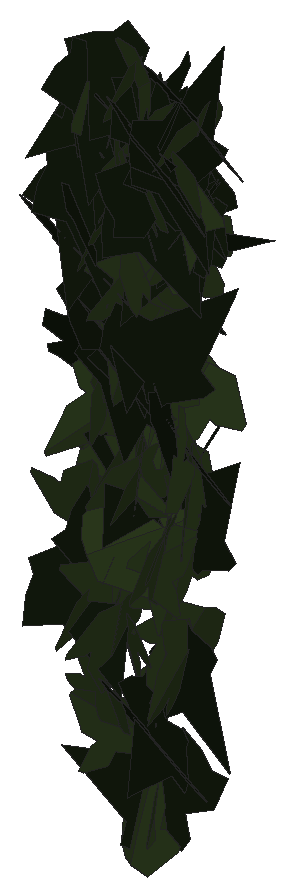
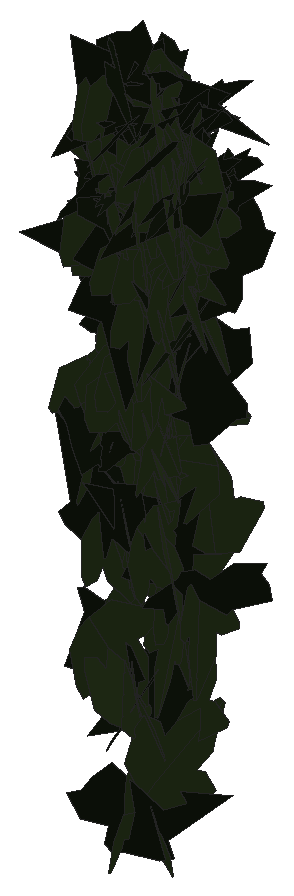
# SketchUp Ruby script. Lengths in inches.
U = 1.inch
M = Sketchup.active_model
def pt(a) = Geom::Point3d.new(a.map { |v| v * U })
def face(e, loops, mat)
  f = e.add_face(loops[0].map { |a| pt(a) })
  loops[1..].each { |l| e.add_face(l.map { |a| pt(a) }).erase! }
  f.material = f.back_material = mat if mat
  f
end
# faces: each face lists its corners as indices into pts; further lists are holes
def faces(e, pts, list, mat = nil) = list.each { |f| face(e, (f[0].is_a?(Array) ? f : [f]).map { |l| l.map { |i| pts[i] } }, mat) }
# xy, xz, yz: faces in a plane at the given z, y or x. An outline is a flat list of corners, or four numbers for a rectangle; further outlines are holes
def ring(l) = l.size == 4 ? [[l[0], l[1]], [l[2], l[1]], [l[2], l[3]], [l[0], l[3]]] : l.each_slice(2).to_a
def flat(e, list, mat, &to3) = list.each { |f| face(e, (f[0].is_a?(Array) ? f : [f]).map { |l| ring(l).map { |u, v| to3.(u, v) } }, mat) }
def xy(e, z, list, mat = nil) = flat(e, list, mat) { |x, y| [x, y, z] }
def xz(e, y, list, mat = nil) = flat(e, list, mat) { |x, z| [x, y, z] }
def yz(e, x, list, mat = nil) = flat(e, list, mat) { |y, z| [x, y, z] }
def lines(e, pts, list) = list.each { |a, b| e.add_line(pt(pts[a]), pt(pts[b])) }
# prism: a flat outline (further loops are holes) pulled along v
def prism(e, loops, v, mat = nil)
  f = face(e, loops, mat); d = Geom::Vector3d.new(v.map { |x| x * U })
  f.pushpull(f.normal.samedirection?(d) ? d.length : -d.length)
end
def box(e, o, s, mat = nil) = prism(e, [[o, [o[0] + s[0], o[1], o[2]], [o[0] + s[0], o[1] + s[1], o[2]], [o[0], o[1] + s[1], o[2]]]], [0, 0, s[2]], mat)
def at(x, y, z, deg = 0) = Geom::Transformation.translation(pt([x, y, z])) * Geom::Transformation.rotation(ORIGIN, Z_AXIS, deg.degrees)
def axes(o, x, y, z) = Geom::Transformation.new([*x, 0, *y, 0, *z, 0, *pt(o).to_a, 1])
def part(name) = M.definitions.add(name)
# library, detail: a bought-in or finely detailed component or shape, given as its bounding box
def library(name, o, s) = part(name).tap { |d| box(d.entities, o, s) }
def detail(e, o, s) = box(e.add_group.entities, o, s)
def put(e, d, t, mat = nil) = e.add_instance(d, t).tap { |i| i.material = mat if mat }
def group(e, t, mat = nil) = e.add_group.tap { |g| g.transformation = t; g.material = mat if mat }.entities
root = M.entities
M.materials.add("efeu1").color = [18, 25, 13]
M.materials.add("efeu2").color = [43, 57, 29]
c1 = part("ivyleaf_9")
p = [[1.54,2.16,1.25],[1.36,2.04,1.19],[-0.21,0.99,0.68],[-0.71,1.11,0.82],[-0.85,0.86,0.67],[-0.8,0.17,0.21],
  [-0.9,-0.01,0.1],[-0.67,-0.16,-0.02],[-0.08,-0.08,-0.05],[-0.03,-0.6,-0.4],[0.65,-0.88,-0.66],[0.83,-0.6,-0.49],
  [1.29,-0.42,-0.43],[1.8125,-0.07,-0.26],[1.21,0.44,0.15]]
faces(c1.entities,p,[[0,1,2,3,4,5,6,7,8,9,10,11,12,13,14]],"efeu1")
c2 = part("ivyleaf_10")
p = [[0,0.5,-0.03],[-0.0625,2.02,-0.43],[-0.19,2.01,-0.46],[-0.54,1.05,-0.29],[-0.52,0.625,-0.18],[-0.83,0.76,-0.28],
  [-1.16,0.64,-0.33],[-1.15,0.33,-0.24],[-0.77,-0.39,0.02],[-0.3,-0.51,0.16],[0.04,-0.48,0.23],[-0.02,2.01,-0.4375],
  [-0.06,2.01,-0.43],[0.04,-0.49,0.23],[0.67,-0.49,0.14],[1.38,0.36,-0.2],[1.375,0.51,-0.24],[0.81,0.65,-0.19],
  [0.62,0.59,-0.15],[0.6,1.09,-0.28],[0.5,1.23,-0.31]]
faces(c2.entities,p,[[0,1,2,3,4,5,6,7,8,9,10],[11,12,0,13,14,15,16,17,18,19,20]],"efeu2")
put(root,c1,axes([25.3,224.21,220.79],[0.23727,-0.27625,0.34262],[0.27235,-0.2136,-0.36083],[0.34573,0.35785,0.04911]))
put(root,c2,axes([25.7,224.74,222.02],[0.25708,-0.41846,-0.09381],[0.00924,0.11476,-0.48656],[0.42874,0.24844,0.06674]))
put(root,c2,axes([25.66,224.67,221.51],[0.33755,0.36179,-0.07186],[-0.05541,-0.04658,-0.49473],[-0.36468,0.34196,0.00865]))
put(root,c2,axes([25.78,224.24,216.53],[0.03843,-0.45656,-0.20019],[-0.0113,0.19994,-0.45815],[0.49839,0.03974,0.00505]))
put(root,c2,axes([25.7,224.72,222.3],[-0.4666,-0.11612,-0.13712],[0.13863,0.01007,-0.48029],[0.1143,-0.48623,0.0228]))
put(root,c1,axes([25.71,223.97,221.64],[0.35482,-0.12342,-0.32996],[-0.28859,0.16676,-0.37271],[0.20204,0.45493,0.04711]))
put(root,c2,axes([25.67,224.15,217.47],[-0.46983,-0.00104,0.17107],[0.17106,-0.00683,0.46978],[0.00136,0.49995,0.00677]))
put(root,c2,axes([25.91,224.8,214.64],[-0.20183,-0.25034,-0.38287],[-0.23596,-0.30154,0.32155],[-0.3919,0.31048,0.00358]))
put(root,c2,axes([25.84,224.67,221.86],[-0.18116,-0.46591,-0.01034],[0.00679,0.00846,-0.49988],[0.46598,-0.18125,0.00326]))
put(root,c1,axes([25.38,224.33,219.46],[0.38974,-0.04686,0.30968],[0.30851,-0.02792,-0.39249],[0.05407,0.49702,0.00715]))
put(root,c2,axes([25.94,224.21,220.41],[0.34987,-0.21771,-0.28319],[-0.23378,0.16016,-0.41194],[0.27007,0.42066,0.01028]))
put(root,c2,axes([25.81,224.68,221.92],[0.16857,-0.46716,0.05788],[0.0158,-0.05583,-0.49662],[0.47046,0.16926,-0.00405]))
put(root,c1,axes([25.57,224.5625,222.11],[0.49853,0.03827,0],[-0.00502,0.0654,-0.49568],[-0.03794,0.49423,0.06559]))
put(root,c1,axes([25.67,224.74,221.89],[0.01646,-0.49973,-0.00146],[0.00007,0.00146,-0.5],[0.49973,0.01646,0.00011]))
put(root,c1,axes([25.77,224.4,221.54],[-0.1775,-0.46732,0.01028],[-0.00411,-0.00944,-0.49989],[0.46742,-0.17755,-0.00049]))
put(root,c2,axes([26.0625,224.37,220.65],[0.23074,-0.22348,-0.38316],[-0.28403,0.25731,-0.32112],[0.34071,0.36585,-0.00821]))
put(root,c1,axes([25.69,224.21,216.82],[-0.06647,-0.41296,-0.27395],[0.05339,0.26882,-0.41819],[0.49268,-0.08485,0.00836]))
put(root,c2,axes([25.81,224.6875,221.76],[-0.46903,-0.09695,-0.14357],[0.14605,0.00158,-0.47819],[0.09317,-0.49051,0.02684]))
put(root,c2,axes([25.77,224.73,221.42],[-0.3733,-0.28773,-0.16692],[0.2134,-0.01468,-0.45194],[0.25517,-0.40865,0.13376]))
put(root,c2,axes([25.6875,224.45,222.45],[0.11924,-0.43016,0.22526],[0.26979,-0.13417,-0.39901],[0.40372,0.21671,0.20011]))
put(root,c2,axes([25.84,224.52,222.52],[0.34144,-0.35958,0.06418],[0.03602,-0.05428,-0.49574],[0.36348,0.34315,-0.01116]))
put(root,c2,axes([25.85,224.91,218.9375],[-0.10473,0.40267,-0.27729],[-0.02921,-0.28823,-0.40752],[-0.48803,-0.06916,0.0839]))
put(root,c1,axes([25.77,224.59,222.75],[-0.08731,-0.4881,0.0643],[0.00023,-0.06534,-0.49571],[0.49232,-0.08653,0.01164]))
put(root,c2,axes([26.02,224.23,215.18],[-0.45975,0.17524,-0.08898],[-0.08678,0.02211,0.49191],[0.17634,0.46776,0.01009]))
put(root,c1,axes([25.6,224.75,222.06],[0.33348,-0.37031,0.04079],[0.05507,-0.00514,-0.49693],[0.36846,0.33592,0.03736]))
put(root,c2,axes([25.95,224.71,222.12],[-0.23348,-0.43652,-0.07027],[0.03089,0.06316,-0.49503],[0.44106,-0.23551,-0.00252]))
put(root,c1,axes([26.13,224.52,222.92],[-0.47502,-0.12045,0.09924],[-0.08474,-0.06791,-0.48806],[0.13106,-0.4805,0.0441]))
put(root,c2,axes([25.99,224.74,220.95],[-0.31643,-0.3736,0.10147],[0.01272,-0.14101,-0.47954],[0.38692,-0.3009,0.09874]))
put(root,c2,axes([25.9,224.59,222.18],[-0.37426,0.32688,-0.05548],[0.0445,-0.03339,-0.4969],[-0.32856,-0.37687,-0.0041]))
put(root,c1,axes([25.79,224.23,221.74],[0.00212,-0.49178,-0.09024],[0.0083,0.09027,-0.49171],[0.49993,0.00059,0.00854]))
put(root,c2,axes([26.03,224.46,216.28],[-0.39846,0.27118,0.133],[-0.10656,0.0798,-0.48195],[-0.28262,-0.41242,-0.0058]))
put(root,c2,axes([26.03,224.61,219.26],[0.05715,0.38173,-0.31783],[-0.17546,-0.28378,-0.3724],[-0.4647,0.1541,0.10153]))
put(root,c2,axes([26.04,224.16,221.4],[0.13555,-0.44192,-0.19062],[-0.06145,0.18052,-0.46221],[0.47734,0.14873,-0.00537]))
put(root,c2,axes([25.875,224.69,220.625],[-0.07184,-0.32443,0.37361],[0.19061,-0.36654,-0.28164],[0.45663,0.10196,0.17634]))
put(root,c1,axes([25.75,224.66,222.44],[0.16645,-0.44634,-0.15191],[0.00711,0.16346,-0.47247],[0.47143,0.15513,0.06077]))
put(root,c2,axes([26.15,224.31,219.05],[-0.13075,-0.18535,0.44559],[-0.1311,-0.43065,-0.2176],[0.46445,-0.17374,0.06402]))
put(root,c2,axes([26.02,224.66,220.2],[0.31523,-0.38728,-0.02535],[-0.01406,0.02123,-0.49935],[0.38786,0.31553,0.00249]))
put(root,c2,axes([26.29,224.14,221.51],[0.18426,-0.04059,-0.46303],[-0.36484,0.29598,-0.17113],[0.28799,0.40093,0.07946]))
put(root,c2,axes([26.03,224.14,219.34],[0.14162,-0.36303,-0.31329],[0.04213,0.33482,-0.36894],[0.47767,0.0781,0.12542]))
put(root,c2,axes([26.12,224.42,217.4375],[0.19341,-0.43236,-0.16017],[-0.07627,0.1413,-0.47352],[0.45473,0.2076,-0.01129]))
put(root,c1,axes([25.79,224.65,219.99],[0.17145,-0.44736,0.1431],[0.06303,-0.12904,-0.47893],[0.46544,0.18226,0.01214]))
put(root,c2,axes([26.0625,224.58,222.9],[0.1817,-0.4647,0.03219],[0.03058,-0.02258,-0.49855],[0.46481,0.18314,0.02022]))
put(root,c2,axes([26.05,224.74,218.85],[0.26099,-0.41098,0.11391],[0.05113,-0.10243,-0.48672],[0.4234,0.26571,-0.01144]))
put(root,c2,axes([26.28,224.39,222.93],[0.25108,-0.19096,-0.38794],[-0.26478,0.28675,-0.31252],[0.34184,0.36237,0.04287]))
put(root,c1,axes([26.08,224.65,222.53],[-0.25924,-0.42666,-0.02758],[0.01099,0.0256,-0.49922],[0.42741,-0.25944,-0.0039]))
put(root,c1,axes([25.86,224.02,220.27],[0.34819,-0.35427,-0.05709],[-0.0222,0.05813,-0.49611],[0.35815,0.34801,0.02475]))
put(root,c2,axes([26.18,224.82,220.94],[-0.40043,-0.28659,0.08674],[0.02348,-0.17444,-0.468],[0.2985,-0.37073,0.15316]))
put(root,c2,axes([26.17,224.73,220.29],[-0.09299,-0.47939,-0.10743],[0.01803,0.10593,-0.48832],[0.49095,-0.09469,-0.00241]))
put(root,c2,axes([25.89,224.58,221.36],[0.35948,0.13645,-0.31962],[0.28213,0.15392,0.38303],[0.20292,-0.45573,0.03367]))
put(root,c2,axes([26.17,224.76,221.61],[0.17502,-0.45573,-0.10809],[0.0004,0.11553,-0.48647],[0.46837,0.17019,0.04081]))
put(root,c2,axes([26.31,224.91,219.25],[-0.45041,-0.10275,0.19125],[-0.13178,-0.22064,-0.4289],[0.17254,-0.43676,0.17167]))
put(root,c1,axes([26.51,224.85,213.83],[-0.09773,0.04002,0.48872],[-0.48866,0.03351,-0.10046],[-0.04079,-0.49727,0.03257]))
put(root,c2,axes([26.1,224.76,217.41],[0.0094,-0.39176,0.31055],[0.13132,-0.29776,-0.3796],[0.48235,0.0887,0.09729]))
put(root,c2,axes([26.1,224.38,222.39],[-0.15869,0.45616,-0.12936],[0.01757,-0.13066,-0.48231],[-0.47382,-0.15762,0.02544]))
put(root,c2,axes([26.21,224.09,216.4375],[-0.01514,-0.4997,-0.00823],[0.00519,0.00808,-0.49991],[0.49974,-0.01522,0.00495]))
put(root,c2,axes([26.31,224.51,222.06],[-0.39405,-0.29531,0.08671],[-0.0673,-0.05479,-0.49241],[0.30033,-0.39974,0.00343]))
put(root,c2,axes([26.21,224.21,216.74],[-0.41114,-0.27656,0.0669],[0.05589,0.03678,0.4955],[-0.279,0.41492,0.00067]))
put(root,c2,axes([26.55,224.61,219.84],[-0.18047,-0.05171,0.46342],[-0.32069,-0.34697,-0.1636],[0.33851,-0.35628,0.09207]))
put(root,c2,axes([26.27,224.65,222.57],[0.46425,-0.17131,-0.0716],[-0.07038,0.01606,-0.49476],[0.17181,0.46946,-0.00921]))
put(root,c2,axes([26.3125,224.3125,218.53],[0.06611,-0.4918,-0.06132],[-0.016,0.05971,-0.49616],[0.49535,0.06756,-0.00784]))
put(root,c2,axes([26.24,224.65,222.1],[0.33104,-0.37078,-0.05415],[0.03145,0.0995,-0.48899],[0.37339,0.32034,0.0892]))
put(root,c1,axes([26.01,224.18,217.08],[-0.07674,-0.00523,0.49405],[0.48554,0.09175,0.07639],[-0.09146,0.49148,-0.009]))
put(root,c1,axes([25.9375,224.61,221.97],[0.03372,-0.20798,0.45344],[0.32731,-0.33375,-0.17742],[0.37648,0.30879,0.11364]))
put(root,c2,axes([26.37,224.54,222.2],[-0.01578,-0.49408,0.07507],[-0.00939,-0.0748,-0.49428],[0.49966,-0.01701,-0.00691]))
put(root,c2,axes([26.23,224.49,213.5],[0.45857,-0.19929,-0.0018],[0.00541,0.00794,0.49991],[-0.19922,-0.4585,0.00944]))
put(root,c2,axes([25.96,224.12,218.16],[-0.11065,0.03724,-0.48618],[0.47188,-0.1174,-0.11639],[-0.12282,-0.48459,-0.00916]))
put(root,c2,axes([26.22,225.02,214.15],[-0.04233,0.24177,-0.43561],[0.07134,-0.42973,-0.24544],[-0.49307,-0.08293,0.00189]))
put(root,c1,axes([26.14,224.5,220.09],[0.00995,-0.44828,0.22123],[0.07125,-0.21774,-0.44442],[0.4948,0.04037,0.05954]))
put(root,c2,axes([26.43,224.58,219.39],[-0.17202,-0.46859,-0.02886],[-0.00517,0.03263,-0.49891],[0.46945,-0.17134,-0.01607]))
put(root,c1,axes([26.47,224.5,220.47],[0.32802,0.24152,-0.28995],[-0.28834,-0.08743,-0.39902],[-0.24344,0.42898,0.08193]))
put(root,c2,axes([26.18,224.32,219.63],[-0.15293,-0.08833,0.46777],[0.33005,-0.37373,0.03733],[0.34305,0.32019,0.17262]))
put(root,c1,axes([26.14,224.32,219.33],[0.02666,-0.39752,0.3021],[0.12055,-0.28846,-0.3902],[0.48452,0.09364,0.08046]))
put(root,c2,axes([26.45,224.13,220.65],[0.01814,-0.49682,0.05327],[0.00433,-0.05314,-0.49715],[0.49965,0.01849,0.00237]))
put(root,c1,axes([26.28,224.47,218.17],[-0.09092,-0.37459,0.31845],[0.0286,-0.32733,-0.37687],[0.49083,-0.05032,0.08095]))
put(root,c2,axes([26.23,224.71,215.35],[0.34456,-0.23834,0.27289],[0.22494,-0.15451,-0.41896],[0.28404,0.41148,0.00075]))
put(root,c2,axes([26.29,225.05,215.45],[-0.06936,-0.35361,-0.34662],[0.10389,-0.35261,0.33893],[-0.48414,-0.02501,0.12239]))
put(root,c1,axes([26.41,224.63,222.39],[-0.30012,-0.39415,-0.06759],[0.04777,0.04857,-0.49534],[0.39704,-0.30378,0.0085]))
put(root,c2,axes([26.56,224.4375,218.85],[-0.48013,0.08039,0.11407],[-0.11357,0.01242,-0.48677],[-0.08109,-0.49334,0.00633]))
put(root,c2,axes([26.55,224,218.34],[0.13461,-0.43756,-0.20106],[-0.04778,0.1956,-0.45767],[0.47916,0.14242,0.01085]))
put(root,c2,axes([26.52,224.14,218.38],[-0.19002,-0.44043,-0.14112],[0.04963,0.13227,-0.47963],[0.45981,-0.19628,-0.00655]))
put(root,c2,axes([26.61,224.93,216.13],[-0.11235,-0.42842,0.23202],[-0.05433,-0.22561,-0.44289],[0.48418,-0.12472,0.00414]))
put(root,c2,axes([26.66,224.82,219.05],[0.046,0.17197,0.46724],[-0.14386,-0.44462,0.17781],[0.47664,-0.1508,0.00857]))
put(root,c1,axes([26.29,224.66,222.6],[0.13884,-0.48021,-0.01097],[0.02291,0.01802,-0.49915],[0.47979,0.1381,0.02701]))
put(root,c1,axes([26.24,224.67,222.03],[0.31547,-0.38254,-0.06436],[0.02627,0.10384,-0.48839],[0.38702,0.30477,0.08561]))
put(root,c2,axes([26.69,224.15,220.83],[-0.33226,-0.31958,0.19358],[-0.13267,-0.14126,-0.46092],[0.34929,-0.35765,0.00907]))
put(root,c1,axes([26.24,224.09,215.43],[0.46067,-0.18896,0.04558],[0.04243,-0.01667,-0.49792],[0.18969,0.46262,0.00068]))
put(root,c2,axes([26.56,224.04,221.98],[-0.41331,0.2809,0.01648],[-0.01397,0.00875,-0.49973],[-0.28104,-0.41354,0.00061]))
put(root,c2,axes([26.26,223.94,217.43],[0.21893,-0.01931,-0.4491],[0.4219,0.18121,0.19789],[0.15513,-0.46561,0.09564]))
put(root,c1,axes([26.71,224.52,222.9],[-0.3847,0.20322,-0.24638],[0.20514,-0.1384,-0.43447],[-0.24479,-0.43537,0.02311]))
put(root,c2,axes([26.82,224.29,222.22],[-0.4244,0.12321,0.23388],[-0.23853,0.01219,-0.43926],[-0.11394,-0.48443,0.04843]))
put(root,c1,axes([26.25,224.46,220.9],[0.29303,-0.0167,0.40479],[0.3956,0.11952,-0.28145],[-0.08736,0.48522,0.08326]))
put(root,c2,axes([26.68,224.59,222.64],[-0.10635,-0.4841,-0.06583],[0.00034,0.06729,-0.49545],[0.48856,-0.10542,-0.01398]))
put(root,c1,axes([26.67,224.73,221.42],[-0.35808,-0.34894,-0.00434],[0.015,-0.00918,-0.49969],[0.34864,-0.35799,0.01704]))
put(root,c2,axes([26.59,224.8,221.4],[0.35095,-0.35543,-0.0224],[0.03811,0.06876,-0.49378],[0.35409,0.34488,0.07536]))
put(root,c2,axes([26.75,224.43,220.84],[-0.40662,-0.27601,0.09209],[-0.06632,-0.06616,-0.49115],[0.28331,-0.41163,0.01719]))
put(root,c1,axes([26.875,224.43,221.36],[-0.19446,0.45494,0.07222],[-0.04503,0.05924,-0.49443],[-0.45843,-0.19879,0.01794]))
put(root,c2,axes([26.65,223.9375,221.17],[-0.08446,0.41354,0.26805],[-0.08796,0.25494,-0.42103],[-0.4849,-0.11828,0.02969]))
put(root,c2,axes([26.47,224.48,219.37],[0.47601,-0.02922,0.15021],[0.14969,-0.01298,-0.47689],[0.03177,0.49898,-0.00361]))
put(root,c1,axes([26.8,224.59,221.46],[-0.48719,-0.08125,-0.07776],[0.07489,0.02351,-0.4938],[0.08389,-0.49279,-0.01074]))
put(root,c1,axes([26.53,224.56,215.04],[-0.02857,-0.33335,0.37157],[-0.00714,-0.37187,-0.33416],[0.49913,-0.0244,0.01648]))
put(root,c2,axes([26.7,224.39,217.59],[0.22499,-0.43979,-0.07721],[-0.02915,0.0718,-0.49396],[0.44557,0.22678,0.00667]))
put(root,c2,axes([26.78,224.72,221.1875],[-0.28062,-0.39019,0.13784],[-0.03965,-0.14043,-0.47823],[0.41192,-0.27933,0.04787]))
put(root,c1,axes([26.44,224.52,222.96],[0.48457,-0.12123,-0.02234],[-0.02144,0.00635,-0.4995],[0.12139,0.48504,0.00095]))
put(root,c2,axes([26.76,224.54,222.2],[-0.02155,-0.41935,0.27145],[0.0191,-0.27219,-0.41898],[0.49917,-0.00769,0.02775]))
put(root,c2,axes([26.75,224.6,217.28],[-0.10002,-0.45831,0.17305],[0.06515,-0.18749,-0.45891],[0.48554,-0.06926,0.09722]))
put(root,c2,axes([26.84,224.72,219.28],[0.31696,0.30725,-0.2348],[-0.21199,-0.11585,-0.43777],[-0.32341,0.37706,0.05683]))
put(root,c1,axes([26.61,224.74,221.78],[0.0298,-0.49026,-0.09357],[-0.00728,0.0933,-0.49116],[0.49906,0.03064,-0.00158]))
put(root,c1,axes([26.43,224.17,222.51],[0.33113,-0.32845,0.1802],[0.12812,-0.12671,-0.4664],[0.35205,0.35505,0.00024]))
put(root,c2,axes([26.8125,224.13,217.51],[0.10794,-0.46302,-0.15479],[0.00453,0.15947,-0.47387],[0.48819,0.1009,0.03862]))
put(root,c1,axes([26.42,224.59,218.8],[0.30343,-0.28317,0.27883],[0.19721,-0.19728,-0.41496],[0.34502,0.36179,-0.00804]))
put(root,c1,axes([26.88,223.99,221.79],[-0.24951,-0.27999,0.33069],[0.21833,0.24837,0.37503],[-0.37427,0.33154,-0.00168]))
put(root,c1,axes([26.64,224.17,221.8125],[0.05338,-0.41871,-0.26802],[-0.00513,0.26908,-0.42139],[0.49712,0.04774,0.02444]))
put(root,c1,axes([26.85,224.03,219.43],[0.29315,-0.14857,-0.37682],[-0.33604,0.1705,-0.32865],[0.22615,0.44593,0.00011]))
put(root,c1,axes([26.65,224.74,217.33],[-0.19768,0.07907,0.4524],[0.33804,-0.30835,0.20161],[0.31088,0.38557,0.06845]))
put(root,c2,axes([26.94,224.5625,222.54],[-0.01103,-0.48598,-0.11705],[-0.00175,0.11711,-0.48609],[0.49988,-0.01031,-0.00428]))
put(root,c1,axes([26.66,224.42,222.27],[0.19495,-0.46043,-0.0014],[0.02503,0.01212,-0.49923],[0.45975,0.19457,0.02777]))
put(root,c2,axes([26.75,224.34,221.68],[0.47254,0.09811,0.13071],[0.12754,0.02872,-0.48261],[-0.1022,0.48944,0.00212]))
put(root,c1,axes([27.09,224.61,218.68],[-0.31636,0.32139,-0.21593],[0.13709,-0.1678,-0.45061],[-0.36211,-0.34431,0.01805]))
put(root,c2,axes([26.81,224.49,216],[0.03961,-0.12152,0.48339],[0.24193,-0.41927,-0.12522],[0.43578,0.24381,0.02559]))
put(root,c1,axes([26.72,223.97,219.7],[-0.14233,-0.0178,0.47898],[0.47912,0.00889,0.1427],[-0.0136,0.4996,0.01453]))
put(root,c1,axes([26.9,224.1875,222.1875],[-0.1153,-0.20284,0.44223],[0.34573,0.28561,0.22114],[-0.34231,0.35677,0.07439]))
put(root,c2,axes([26.68,224.2,217.28],[0.24682,-0.20231,-0.3849],[0.32058,-0.21435,0.31825],[-0.29378,-0.40388,0.0239]))
put(root,c2,axes([27.06,224.04,218.36],[0.35584,-0.27587,0.21742],[-0.1751,0.12898,0.45023],[-0.3045,-0.39656,-0.00482]))
put(root,c1,axes([26.71,224.59,215.95],[-0.08899,-0.05997,-0.48835],[0.47671,0.11231,-0.10066],[0.12177,-0.48352,0.03719]))
put(root,c2,axes([26.94,224.59,218.33],[-0.11147,0.3666,-0.32121],[0.03465,-0.32271,-0.38034],[-0.48618,-0.10705,0.04654]))
